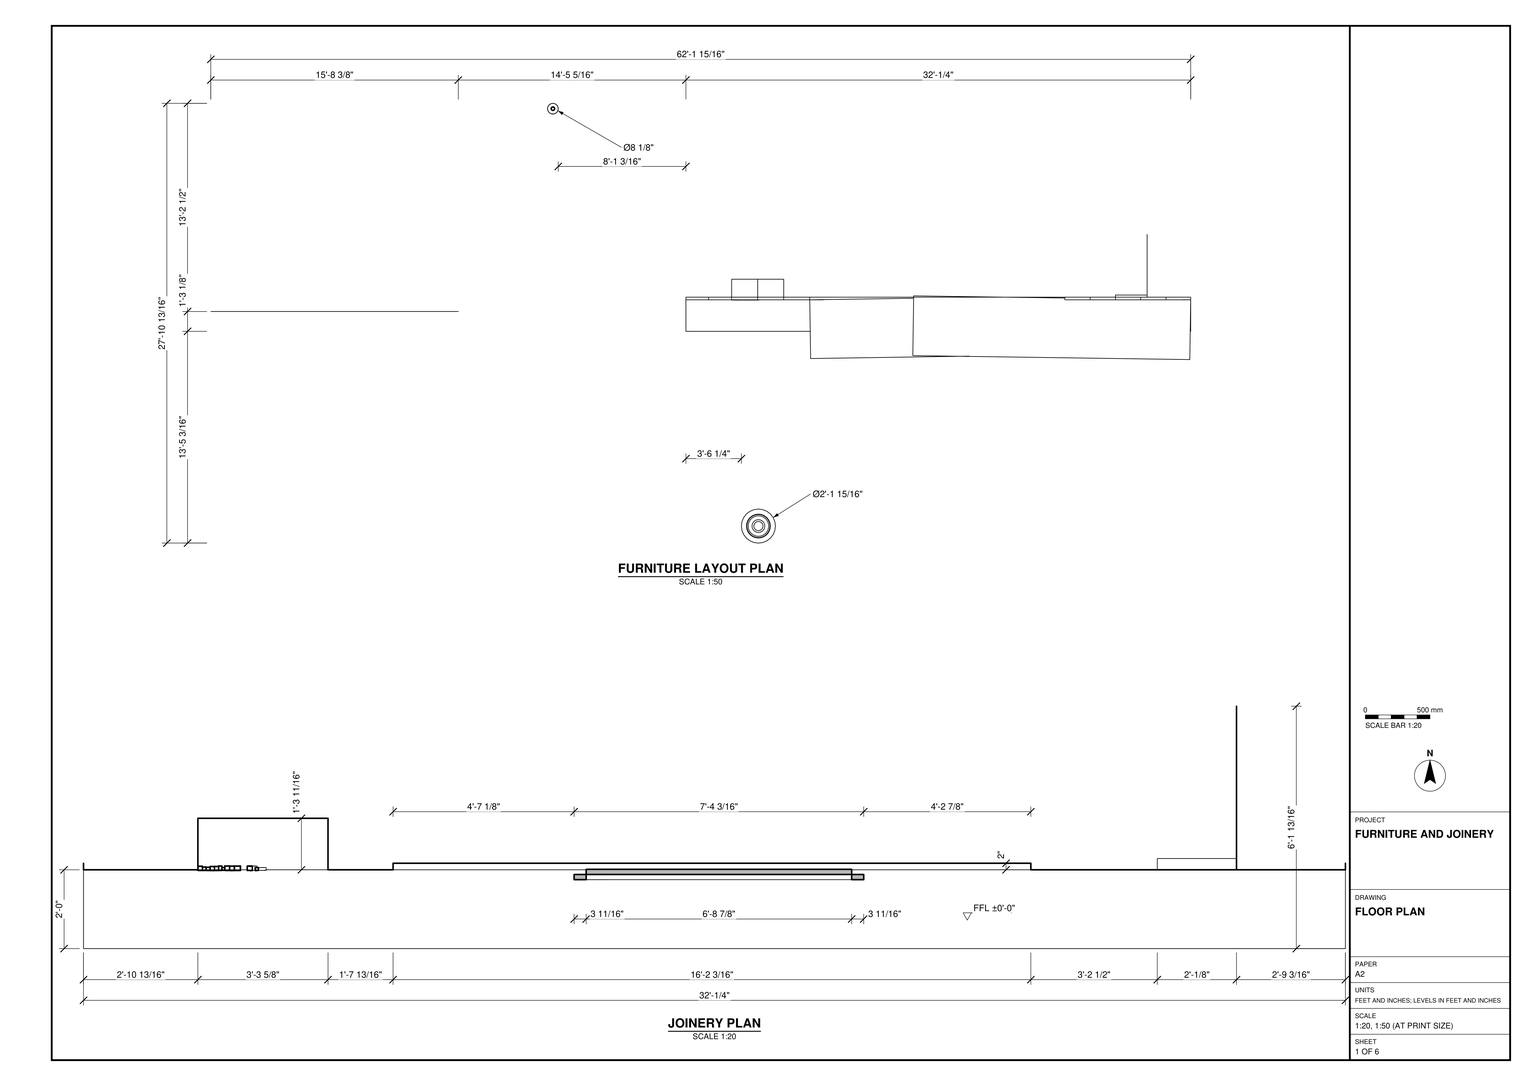
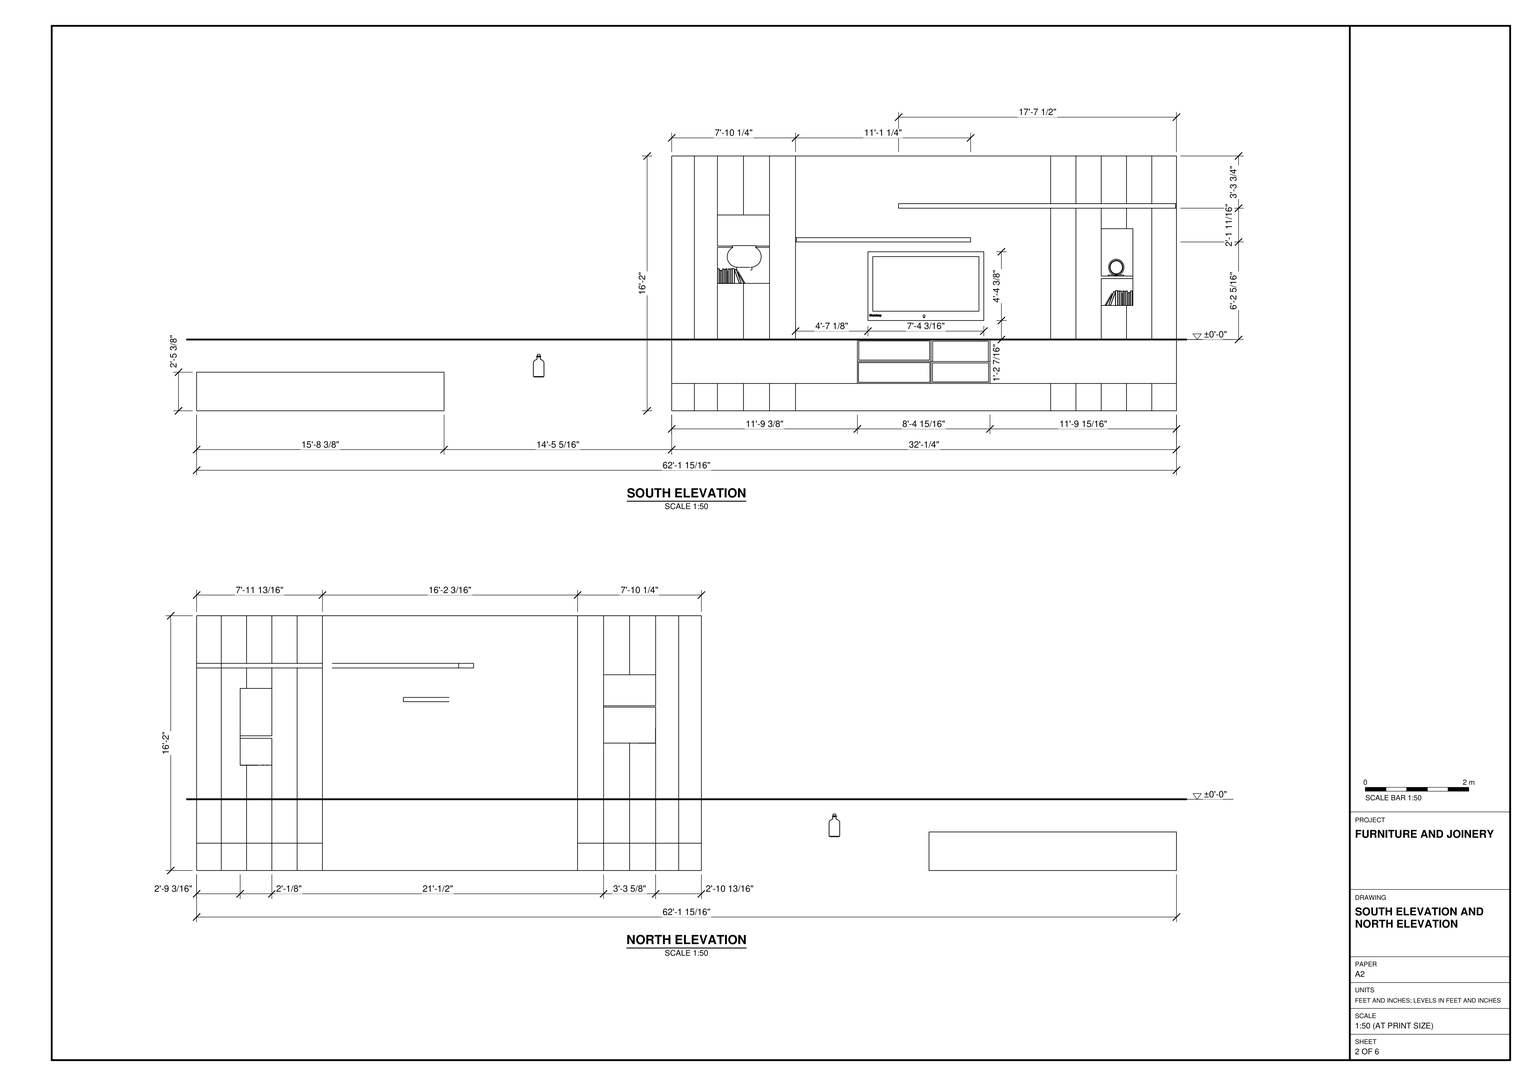
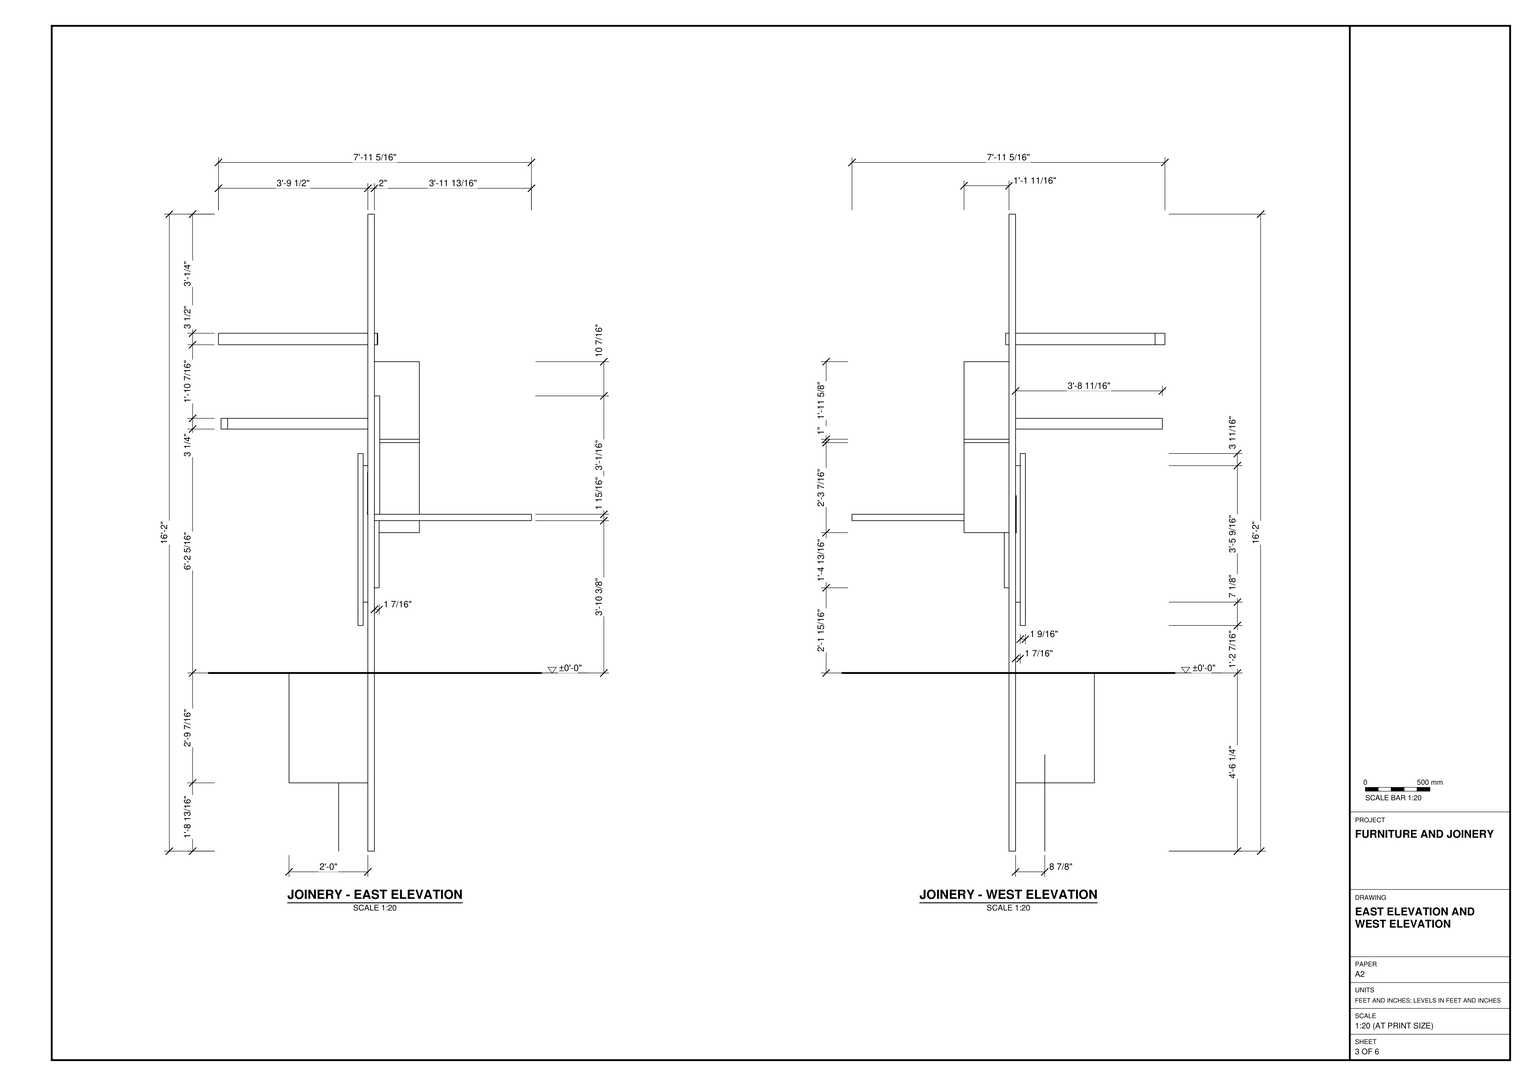
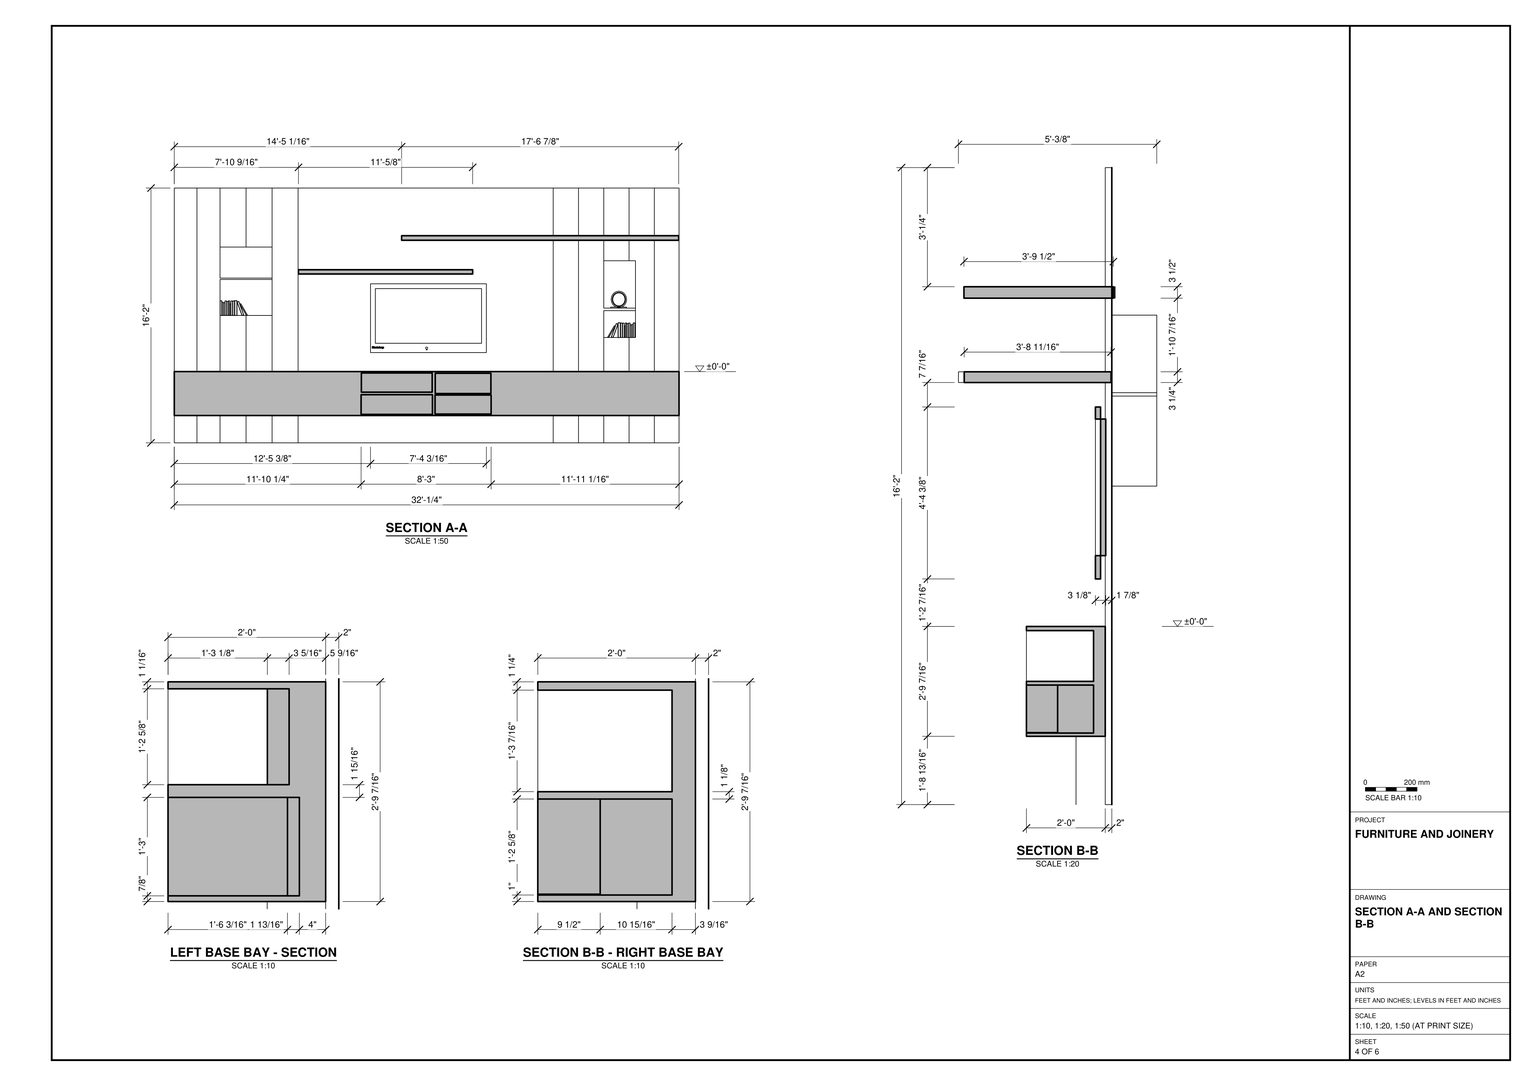
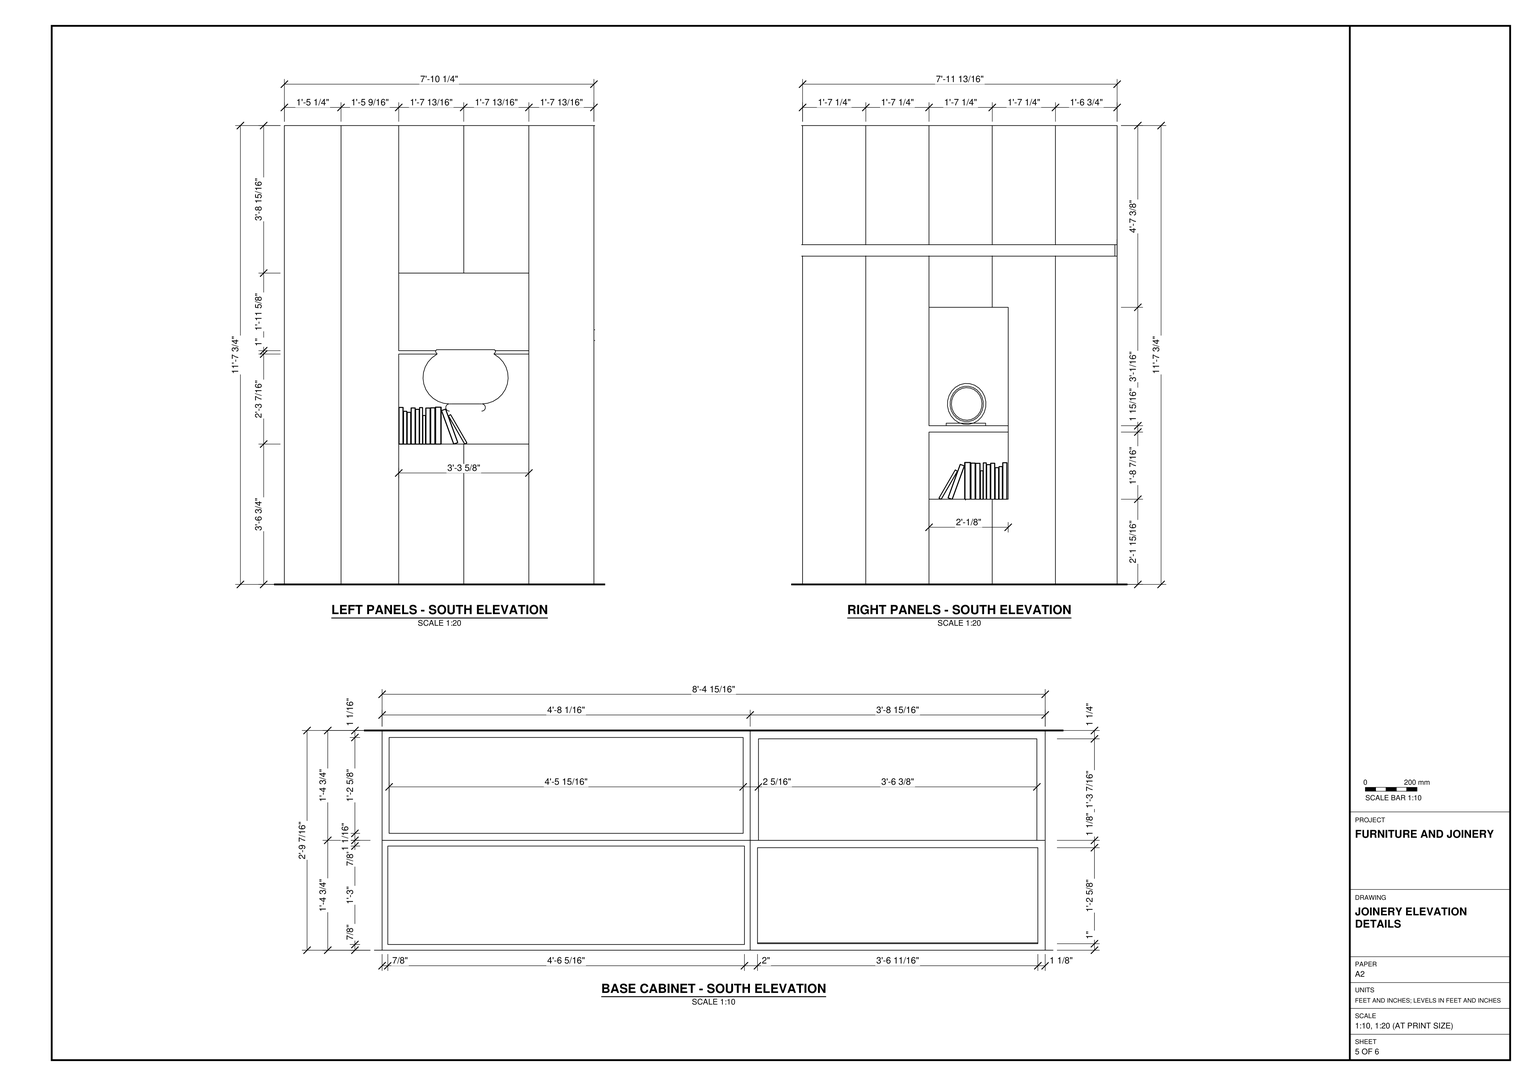
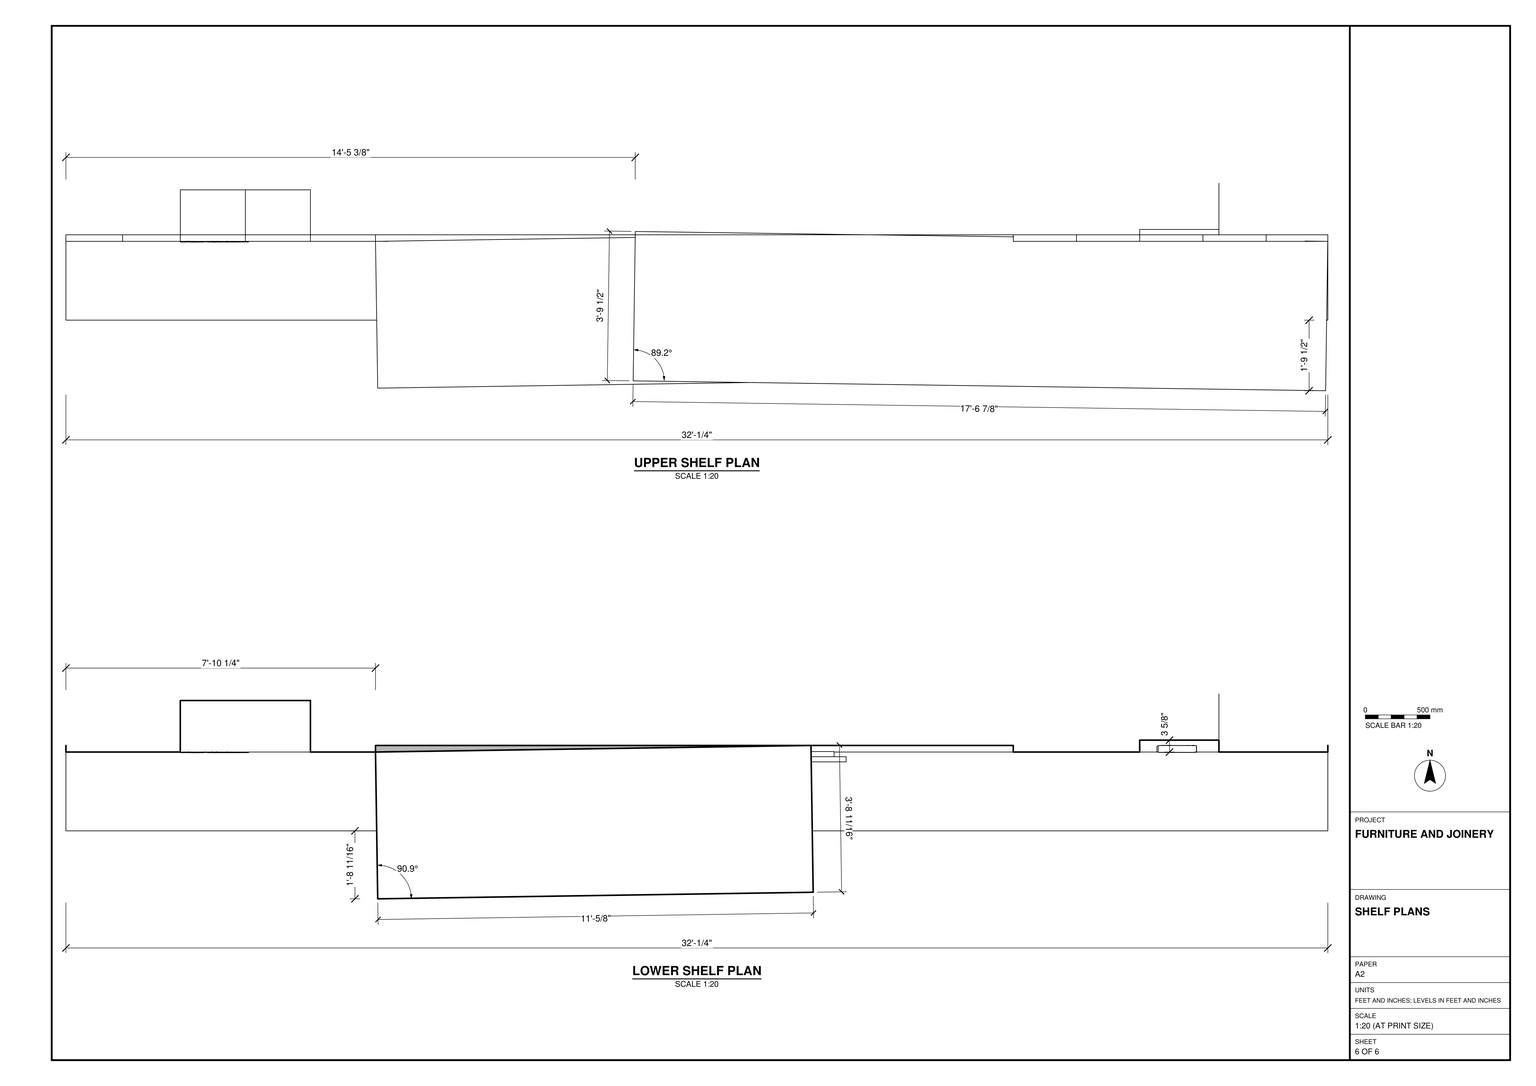
Build the TV wall and the separate items shown in task_files/diagram_01.pdf. Work in feet and inches. The complete layout measures 62'-1 15/16" along X, 27'-10 13/16" along Y and 16'-2" along Z. Use the single level ±0'-0" at the top of the low cabinet run; the backing continues below this level.

Use the joinery plan to set out the 32'-1/4" main run. Form the broad central TV panel and the narrower vertical panels at each end. Match the display recesses in the south elevation, and place the TV above the central storage compartments. Model the two projecting shelves at their different heights: the lower shelf starts at the left edge of the TV panel, while the longer upper shelf reaches the right end of the unit. Use the end elevations to set the backing thickness, cabinet depth and projections on both faces.

Follow the furniture layout plan to position the separate rectangular panel, bottle and pot. Decor and loose items may be any suitable library components. Keep each furniture or joinery piece in a separate group or component, with repeated parts made as components. Save one SketchUp model as output_files/panelled_tv_wall_with_shelves_and_low_storage.skp.

# SketchUp Ruby script. Lengths in inches.
U = 1.inch
M = Sketchup.active_model
def pt(a) = Geom::Point3d.new(a.map { |v| v * U })
def face(e, loops, mat)
  f = e.add_face(loops[0].map { |a| pt(a) })
  loops[1..].each { |l| e.add_face(l.map { |a| pt(a) }).erase! }
  f.material = f.back_material = mat if mat
  f
end
# faces: each face lists its corners as indices into pts; further lists are holes
def faces(e, pts, list, mat = nil) = list.each { |f| face(e, (f[0].is_a?(Array) ? f : [f]).map { |l| l.map { |i| pts[i] } }, mat) }
# xy, xz, yz: faces in a plane at the given z, y or x. An outline is a flat list of corners, or four numbers for a rectangle; further outlines are holes
def ring(l) = l.size == 4 ? [[l[0], l[1]], [l[2], l[1]], [l[2], l[3]], [l[0], l[3]]] : l.each_slice(2).to_a
def flat(e, list, mat, &to3) = list.each { |f| face(e, (f[0].is_a?(Array) ? f : [f]).map { |l| ring(l).map { |u, v| to3.(u, v) } }, mat) }
def xy(e, z, list, mat = nil) = flat(e, list, mat) { |x, y| [x, y, z] }
def xz(e, y, list, mat = nil) = flat(e, list, mat) { |x, z| [x, y, z] }
def yz(e, x, list, mat = nil) = flat(e, list, mat) { |y, z| [x, y, z] }
def lines(e, pts, list) = list.each { |a, b| e.add_line(pt(pts[a]), pt(pts[b])) }
# prism: a flat outline (further loops are holes) pulled along v
def prism(e, loops, v, mat = nil)
  f = face(e, loops, mat); d = Geom::Vector3d.new(v.map { |x| x * U })
  f.pushpull(f.normal.samedirection?(d) ? d.length : -d.length)
end
def box(e, o, s, mat = nil) = prism(e, [[o, [o[0] + s[0], o[1], o[2]], [o[0] + s[0], o[1] + s[1], o[2]], [o[0], o[1] + s[1], o[2]]]], [0, 0, s[2]], mat)
def at(x, y, z, deg = 0) = Geom::Transformation.translation(pt([x, y, z])) * Geom::Transformation.rotation(ORIGIN, Z_AXIS, deg.degrees)
def axes(o, x, y, z) = Geom::Transformation.new([*x, 0, *y, 0, *z, 0, *pt(o).to_a, 1])
def part(name) = M.definitions.add(name)
# library, detail: a bought-in or finely detailed component or shape, given as its bounding box
def library(name, o, s) = part(name).tap { |d| box(d.entities, o, s) }
def detail(e, o, s) = box(e.add_group.entities, o, s)
def put(e, d, t, mat = nil) = e.add_instance(d, t).tap { |i| i.material = mat if mat }
def group(e, t, mat = nil) = e.add_group.tap { |g| g.transformation = t; g.material = mat if mat }.entities
root = M.entities
c1 = part("Sketchup\#2")
xy(c1.entities,0.02,[[[19.26,0,19.26,3.48,19.89,3.48,19.89,3.11,20.03,3.29,20.21,3.42,20.43,3.51,20.67,3.54,20.88,3.52,21.08,3.45,21.26,3.35,21.42,3.2,21.55,3.01,21.65,2.78,21.71,2.53,21.73,2.24,21.71,1.9375,21.65,1.67,21.55,1.45,21.42,1.25,21.25,1.1,21.08,0.99,20.88,0.92,20.67,0.9,20.47,0.92,20.29,0.99,20.11,1.1,19.93,1.27,19.93,0],[20.5,1.43,20.72,1.48,20.89,1.62,20.96,1.73,21.01,1.87,21.05,2.23,21.01,2.58,20.96,2.71,20.89,2.82,20.71,2.97,20.49,3.01,20.27,2.97,20.09,2.82,20.02,2.72,19.96,2.59,19.92,2.26,19.97,1.89,20.02,1.75,20.09,1.64,20.28,1.48,20.39,1.45]],[1.61,0.9,1.3,0.92,1.03,0.97,0.8,1.07,0.6,1.2,0.44,1.375,0.32,1.58,0.23,1.82,0.18,2.09,0.86,2.16,0.95,1.86,1.11,1.65,1.33,1.53,1.62,1.49,1.92,1.53,2.13,1.64,2.26,1.79,2.31,1.97,2.29,2.09,2.23,2.18,2.13,2.26,1.98,2.33,1.42,2.49,0.94,2.64,0.76,2.73,0.62,2.83,0.48,2.98,0.38,3.15,0.32,3.33,0.3,3.53,0.34,3.79,0.45,4.03,0.64,4.23,0.89,4.38,1.2,4.47,1.57,4.5,1.88,4.49,2.15,4.43,2.375,4.34,2.5625,4.22,2.71,4.06,2.8125,3.88,2.88,3.68,2.91,3.45,2.21,3.42,2.13,3.65,2.01,3.8,1.83,3.89,1.57,3.92,1.29,3.89,1.09,3.8,1,3.7,0.97,3.58,1,3.46,1.08,3.37,1.31,3.25,1.73,3.13,2.17,3.01,2.48,2.88,2.7,2.73,2.87,2.53,2.97,2.28,3.01,1.97,2.97,1.68,2.84,1.41,2.64,1.1875,2.37,1.03,2.03,0.93],[[7.33,0.9,7.02,0.93,6.76,1.01,6.54,1.15,6.36,1.33,6.25,1.52,6.17,1.72,6.125,1.95,6.11,2.2,6.13,2.5,6.1875,2.76,6.29,2.99,6.44,3.1875,6.61,3.34,6.81,3.45,7.02,3.52,7.26,3.54,7.53,3.52,7.77,3.45,7.98,3.33,8.15,3.17,8.3,2.96,8.39,2.7,8.45,2.39,8.46,2.03,6.79,2.03,6.84,1.77,6.95,1.57,7.13,1.44,7.34,1.4,7.48,1.42,7.6,1.49,7.7,1.6,7.76,1.76,8.43,1.65,8.26,1.33,8.15,1.2,8.02,1.09,7.88,1.01,7.71,0.95],[6.8,2.4375,7.8,2.4375,7.76,2.69,7.65,2.88,7.49,2.99,7.31,3.03,7.11,2.99,6.94,2.87,6.84,2.68]],[9.69,0.9,9.52,0.92,9.37,0.96,9.24,1.03,9.16,1.12,9.1,1.23,9.0625,1.38,9.04,1.85,9.04,2.95,8.73,2.95,8.73,3.48,9.04,3.48,9.04,3.99,9.71,4.375,9.71,3.48,10.17,3.48,10.17,2.95,9.71,2.95,9.71,1.93,9.72,1.57,9.78,1.49,9.9,1.46,10.16,1.52,10.22,1,9.97,0.93],[11.69,0.9,11.43,0.92,11.2,0.99,10.99,1.1,10.8125,1.25,10.67,1.44,10.56,1.67,10.5,1.93,10.48,2.22,10.5,2.51,10.57,2.78,10.67,3,10.8125,3.19,10.99,3.35,11.2,3.45,11.4375,3.52,11.71,3.54,11.93,3.53,12.12,3.49,12.29,3.43,12.44,3.34,12.57,3.23,12.67,3.09,12.76,2.93,12.83,2.74,12.17,2.62,12.12,2.79,12.02,2.92,11.89,2.99,11.72,3.02,11.49,2.97,11.32,2.84,11.25,2.74,11.21,2.61,11.17,2.27,11.21,1.88,11.25,1.74,11.32,1.63,11.5,1.49,11.73,1.45,11.9,1.47,12.04,1.56,12.14,1.7,12.21,1.93,12.86,1.82,12.8,1.6,12.71,1.42,12.6,1.26,12.47,1.13,12.3125,1.03,12.13,0.96,11.93,0.92],
  [17.13,0.9,16.89,0.93,16.68,1.01,16.5,1.15,16.39,1.33,16.32,1.57,16.3,1.89,16.3,3.48,16.96,3.48,16.96,2.32,16.97,1.89,17,1.67,17.05,1.5625,17.13,1.48,17.24,1.43,17.38,1.41,17.54,1.44,17.6875,1.51,17.8,1.61,17.875,1.74,17.91,1.98,17.92,2.42,17.92,3.48,18.59,3.48,18.59,0.96,17.97,0.96,17.97,1.34,17.8125,1.16,17.61,1.02,17.38,0.93],[3.57,0.96,3.57,4.44,4.24,4.44,4.24,2.6,5.02,3.48,5.84,3.48,4.98,2.5625,5.91,0.96,5.19,0.96,4.55,2.09,4.24,1.77,4.24,0.96],[13.33,0.96,13.33,4.44,14,4.44,14,3.16,14.17,3.33,14.36,3.45,14.56,3.52,14.77,3.54,14.99,3.52,15.19,3.46,15.35,3.36,15.47,3.24,15.55,3.1,15.6,2.94,15.63,2.44,15.63,0.96,14.96,0.96,14.96,2.62,14.93,2.8,14.875,2.89,14.79,2.97,14.68,3.01,14.55,3.03,14.39,3.01,14.25,2.95,14.14,2.85,14.0625,2.71,14.02,2.5,14,2.22,14,0.96]])
c2 = part("On\#1")
xy(c2.entities,0,[[[0.17,0,0.13,0.01,0.07,0.05,0.05,0.08,0.04,0.12,0.03,0.15,0.02,0.2,0.04,0.3,0.06,0.33,0.1,0.37,0.13,0.38,0.17,0.4,0.25,0.4,0.29,0.39,0.35,0.35,0.37,0.32,0.39,0.28,0.4,0.24,0.4,0.16,0.39,0.12,0.37,0.08,0.35,0.05,0.29,0.01,0.25,0],[0.1875,0.07,0.23,0.07,0.29,0.1,0.3,0.12,0.3125,0.14,0.32,0.17,0.32,0.23,0.3125,0.26,0.3,0.28,0.29,0.3,0.26,0.33,0.17,0.33,0.15,0.31,0.13,0.3,0.11,0.26,0.11,0.23,0.1,0.2,0.11,0.17,0.11,0.14,0.13,0.1,0.17,0.08]],[0.46,0.01,0.46,0.29,0.53,0.29,0.53,0.25,0.55,0.27,0.59,0.29,0.64,0.29,0.67,0.28,0.68,0.27,0.7,0.26,0.7,0.25,0.71,0.23,0.71,0.01,0.64,0.01,0.64,0.21,0.62,0.23,0.61,0.23,0.59,0.24,0.58,0.23,0.56,0.23,0.55,0.21,0.54,0.2,0.53,0.17,0.53,0.01]])
c3 = part("tv")
xy(c3.entities,0,[[0,0,88.1875,1.57]])
xy(c3.entities,7.1,[[3.67,0,84.52,3.15]])
xy(c3.entities,48.69,[[3.67,0,84.52,3.15]])
xy(c3.entities,52.36,[[0,0,88.1875,1.57]])
xz(c3.entities,0,[[[0,0,88.1875,52.36],[3.67,7.1,84.52,48.69],[42.68,2.67,42.48,2.71,42.29,2.8,42.14,2.9375,42.02,3.11,41.96,3.3,41.94,3.51,41.98,3.71,42.07,3.9,42.21,4.05,42.38,4.16,42.57,4.23,42.78,4.24,42.98,4.2,43.16,4.11,43.32,3.98,43.43,3.81,43.5,3.61,43.51,3.41,43.47,3.21,43.38,3.02,43.25,2.87,43.08,2.75,42.88,2.6875]],[42.68,2.67,42.88,2.6875,43.08,2.75,43.25,2.87,43.38,3.02,43.47,3.21,43.51,3.41,43.5,3.61,43.43,3.81,43.32,3.98,43.16,4.11,42.98,4.2,42.78,4.24,42.57,4.23,42.38,4.16,42.21,4.05,42.07,3.9,41.98,3.71,41.94,3.51,41.96,3.3,42.02,3.11,42.14,2.9375,42.29,2.8,42.48,2.71]])
xz(c3.entities,1.57,[[0,0,88.1875,52.36]])
xz(c3.entities,3.15,[[3.67,7.1,84.52,48.69]])
yz(c3.entities,0,[[0,0,1.57,52.36]])
yz(c3.entities,3.67,[[0,7.1,3.15,48.69]])
yz(c3.entities,84.52,[[0,7.1,3.15,48.69]])
yz(c3.entities,88.1875,[[0,0,1.57,52.36]])
put(c3.entities,c1,axes([1.05,0,2.87],[0.4189,0,0],[0,0,0.4189],[0,-1,0]))
put(c3.entities,c2,axes([42.375,0,2.01],[1,0,0],[0,0,1],[0,-1,0]))
c4 = library("Group145\#1",[5.875,6.46,9.56],[20.8,10.13,11.36])
c5 = library("Clock",[22.14,2.03,0],[115.17,46.93,115.16])
c6 = library("pot",[-0.85,-7.22,0],[25.92,25.92,18.7])
c7 = library("bottle",[-29.625,20.67,-4.625],[8.16,8.15,17.3])
xy(root,37.53,[[560.33,21.49,602.71,41.93]])
xy(root,38.59,[[504.09,21.49,558,36.62]])
xy(root,52.99,[[560.33,21.49,602.71,41.93]])
xy(root,53.19,[[504.09,21.49,558,36.62]])
xy(root,154.22,[[745.24,0,534.39,3.01,535.04,48.5,546.41,48.34,745.89,45.49]])
xy(root,157.71,[[745.24,0,745.89,45.49,546.41,48.34,535.04,48.5,534.39,3.01]])
xz(root,21.49,[[361.67,20.8,503.02,54.25],[[503.02,20.8,559.0625,37.53],[503.89,21.67,558.19,36.66]],[[559.0625,20.8,603.98,37.53],[560.18,21.92,602.86,36.41]],[603.98,20.8,745.92,54.25],[503.89,21.67,558.19,36.66],
  [560.18,21.92,602.86,36.41],[[503.02,37.53,559.0625,54.25],[504.09,38.59,558,53.19]],[559.0625,37.53,560.33,37.53,560.33,52.99,602.71,52.99,602.71,37.53,603.98,37.53,603.98,54.25,559.0625,54.25]])
xz(root,36.59,[[0,0,188.375,29.375]])
xz(root,36.62,[[504.09,38.59,558,53.19]])
xz(root,41.93,[[560.33,37.53,602.71,52.99]])
xz(root,45.49,[[745.89,154.22,745.92,159.33]])
yz(root,504.09,[[21.49,38.59,36.62,53.19]])
yz(root,558,[[21.49,38.59,36.62,53.19]])
yz(root,560.33,[[21.49,37.53,41.93,52.99]])
yz(root,602.71,[[21.49,37.53,41.93,52.99]])
p = [[745.24,0,154.22],[745.24,0,157.71],[534.39,3.01,157.71],[534.39,3.01,154.22],[745.89,45.49,154.22],[745.89,45.49,157.71],
  [535.04,48.5,154.22],[535.04,48.5,157.71],[546.41,48.34,154.22],[546.41,48.34,157.71],[546.41,48.34,157.08]]
faces(root,p,[[0,1,2,3],[0,4,5,1],[6,7,2,3],[8,4,5,9,10],[6,8,10,9,7]])
put(root,c3,at(511.05,42.49,68.72))
put(root,c4,axes([685.74,45.1,70.53],[1,0,0],[0,0.14,0],[0,0,1]))
put(root,c5,axes([691.54,45.27,102.58],[0.1049,0,0],[0,0.04616,0],[0,0,0.11167]))
put(root,c4,axes([423.17,44.35,87.36],[-1,0,0],[0,0.14,0],[0,0,1]))
put(root,c6,at(404.74,-132.49,107.04))
put(root,c7,at(285.94,166.26,30.34))
g1 = group(root,at(361.67,47.49,0))
xy(g1,0,[[0,-2,17.26,0],[17.26,-2,34.83,0],[34.83,-2,54.64,0],[54.64,-2,74.45,0],[74.45,-2,94.26,0],
  [288.47,-2,307.72,0],[307.72,-2,326.97,0],[326.97,-2,346.22,0],[346.22,-2,365.47,0],[365.47,-2,384.25,0]])
xy(g1,80.2,[[326.97,-2,351.09,1.4375]])
xy(g1,96.99,[[34.83,-2,74.45,13.6875]])
xy(g1,100.65,[[326.97,-2,351.09,1.4375]])
xy(g1,102.58,[[326.97,-2,351.09,1.625]])
xy(g1,124.4,[[34.83,-2,74.45,13.6875]])
xy(g1,125.43,[[34.83,-2,74.45,13.6875]])
xy(g1,138.64,[[326.97,-2,351.09,1.625]])
xy(g1,149.06,[[34.83,-2,54.64,13.6875],[54.64,-2,74.45,13.6875]])
xy(g1,193.99,[[0,-2,17.26,0],[17.26,-2,34.83,0],[34.83,-2,54.64,0],[54.64,-2,74.45,0],[74.45,-2,94.26,0],
  [288.47,-2,307.72,0],[307.72,-2,326.97,0],[326.97,-2,346.22,0],[346.22,-2,365.47,0],[365.47,-2,384.25,0]])
xz(g1,-2,[[0,0,17.26,193.99],[17.26,0,34.83,0,34.83,124.4,74.45,124.4,74.45,125.43,34.83,125.43,34.83,193.99,17.26,193.99],[34.83,0,54.64,96.99],[54.64,0,74.45,96.99],[74.45,0,94.26,193.99],
  [288.47,0,307.72,193.99],[307.72,0,326.97,0,326.97,100.65,351.09,100.65,351.09,102.58,326.97,102.58,326.97,193.99,307.72,193.99],[326.97,0,346.22,80.2],[346.22,0,365.47,0,365.47,193.99,346.22,193.99,346.22,138.64,351.09,138.64,351.09,80.2,346.22,80.2],[365.47,0,384.25,193.99],
  [326.97,138.64,346.22,193.99],[34.83,149.06,54.64,193.99],[54.64,149.06,74.45,193.99]])
xz(g1,0,[[94.26,0,288.47,193.99]])
xz(g1,1.4375,[[326.97,80.2,351.09,100.65]])
xz(g1,1.625,[[326.97,102.58,351.09,138.64]])
xz(g1,13.6875,[[34.83,96.99,74.45,124.4],[34.83,125.43,74.45,149.06]])
yz(g1,0,[[-2,0,0,193.99]])
yz(g1,34.83,[[-2,96.99,13.6875,124.4],[-2,125.43,13.6875,149.06]])
yz(g1,74.45,[[-2,96.99,13.6875,124.4],[-2,124.4,13.6875,125.43],[-2,125.43,13.6875,149.06]])
yz(g1,94.26,[[-2,0,0,193.99]])
yz(g1,288.47,[[-2,0,0,193.99]])
yz(g1,326.97,[[-2,80.2,1.4375,100.65],[-2,102.58,1.625,138.64]])
yz(g1,351.09,[[-2,80.2,1.4375,100.65],[-2,100.65,47.8125,102.58],[-2,102.58,1.625,138.64]])
yz(g1,384.25,[[-2,0,0,193.99]])
g2 = group(root,at(455.93,0.79,128.54))
prism(g2,[[[0,44.7,0],[132.6,46.7,0],[133.28,2,0],[0.67,0,0]]],[0,0,3.26])
g3 = group(root,at(361.67,21.49,20.8))
xy(g3,0,[[0,0,384.25,24]])
xy(g3,0.87,[[142.23,0,196.53,18.1875],[142.23,18.1875,196.53,20]])
xy(g3,0.99,[[198.51,0,241.2,20.4375]])
xy(g3,1.12,[[198.51,0,241.2,9.5]])
xy(g3,15.61,[[198.51,0,241.2,9.5],[198.51,9.5,241.2,20.4375]])
xy(g3,15.86,[[142.23,0,196.53,18.1875],[142.23,18.1875,196.53,20]])
xy(g3,16.73,[[198.66,0,241.05,20.4375]])
xy(g3,17.79,[[142.42,0,196.33,18.4375]])
xy(g3,32.1875,[[198.66,0,241.05,20.4375]])
xy(g3,32.39,[[142.42,0,196.33,18.4375]])
xy(g3,33.45,[[0,0,384.25,24]])
xz(g3,0,[[0,0,141.36,33.45],[[141.36,0,197.4,16.73],[142.23,0.87,196.53,15.86]],[[197.4,0,384.25,0,384.25,33.45,242.3125,33.45,242.3125,16.73,197.4,16.73],[198.51,0.99,241.2,15.61]],[198.51,0.99,241.2,1.12],[[141.36,16.73,197.4,33.45],[142.42,17.79,196.33,32.39]],
  [197.4,16.73,198.66,16.73,198.66,32.1875,241.05,32.1875,241.05,16.73,242.3125,16.73,242.3125,33.45,197.4,33.45]])
xz(g3,9.5,[[198.51,1.12,241.2,15.61]])
xz(g3,18.1875,[[142.23,0.87,196.53,15.86]])
xz(g3,18.4375,[[142.42,17.79,196.33,32.39]])
xz(g3,20,[[142.23,0.87,196.53,15.86]])
xz(g3,20.4375,[[198.51,0.99,241.2,15.61],[198.66,16.73,241.05,32.1875]])
xz(g3,24,[[0,0,384.25,33.45]])
yz(g3,0,[[0,0,24,33.45]])
yz(g3,142.23,[[0,0.87,18.1875,15.86],[18.1875,0.87,20,15.86]])
yz(g3,142.42,[[0,17.79,18.4375,32.39]])
yz(g3,196.33,[[0,17.79,18.4375,32.39]])
yz(g3,196.53,[[0,0.87,18.1875,15.86],[18.1875,0.87,20,15.86]])
yz(g3,198.51,[[0,0.99,20.4375,0.99,20.4375,15.61,9.5,15.61,9.5,1.12,0,1.12],[0,1.12,9.5,15.61]])
yz(g3,198.66,[[0,16.73,20.4375,32.1875]])
yz(g3,241.05,[[0,16.73,20.4375,32.1875]])
yz(g3,241.2,[[0,0.99,0,1.12,9.5,1.12,9.5,15.61,20.4375,15.61,20.4375,0.99],[0,1.12,9.5,15.61]])
yz(g3,384.25,[[0,0,24,33.45]])
